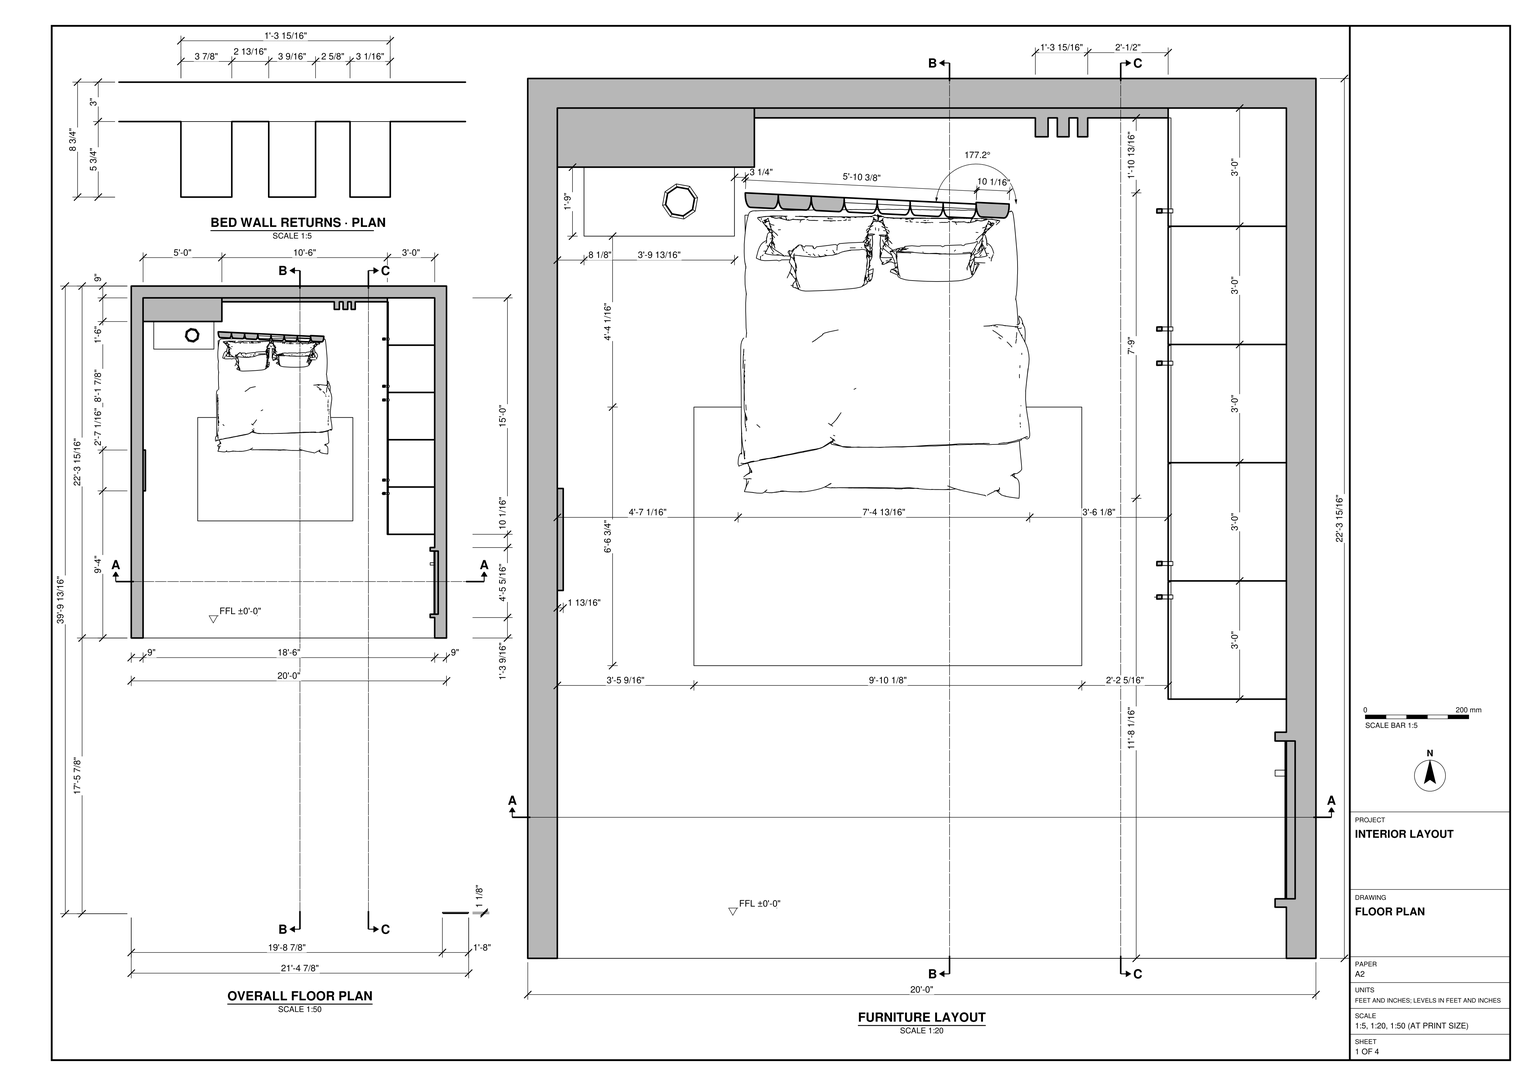
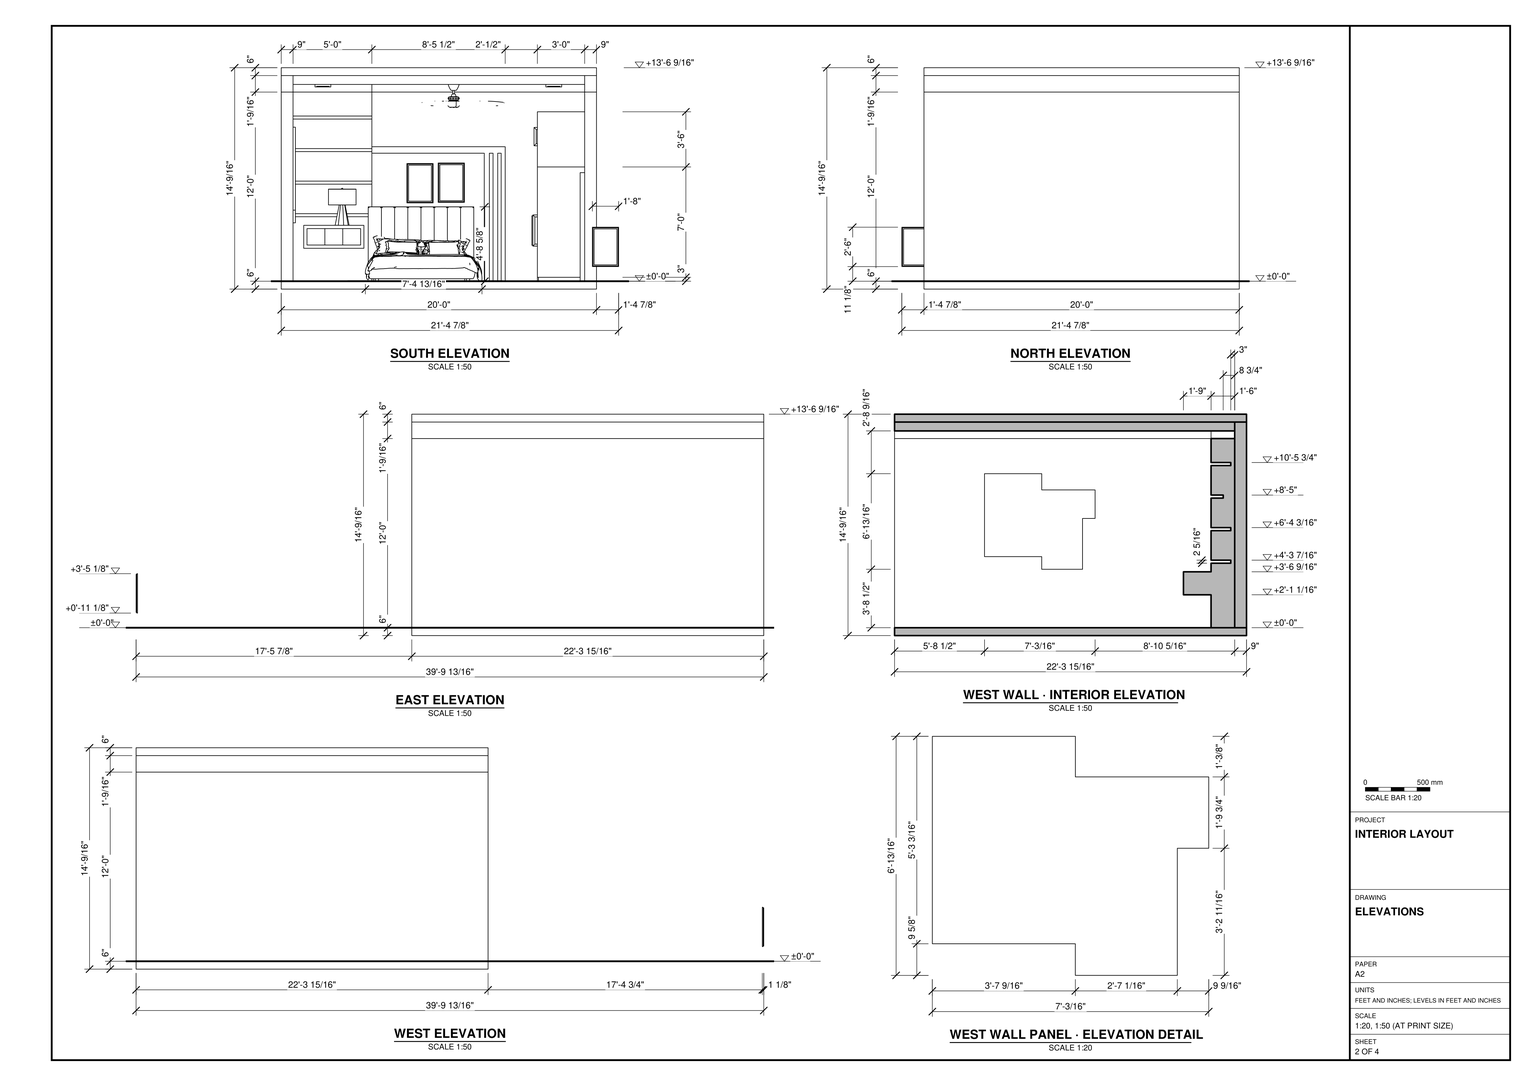
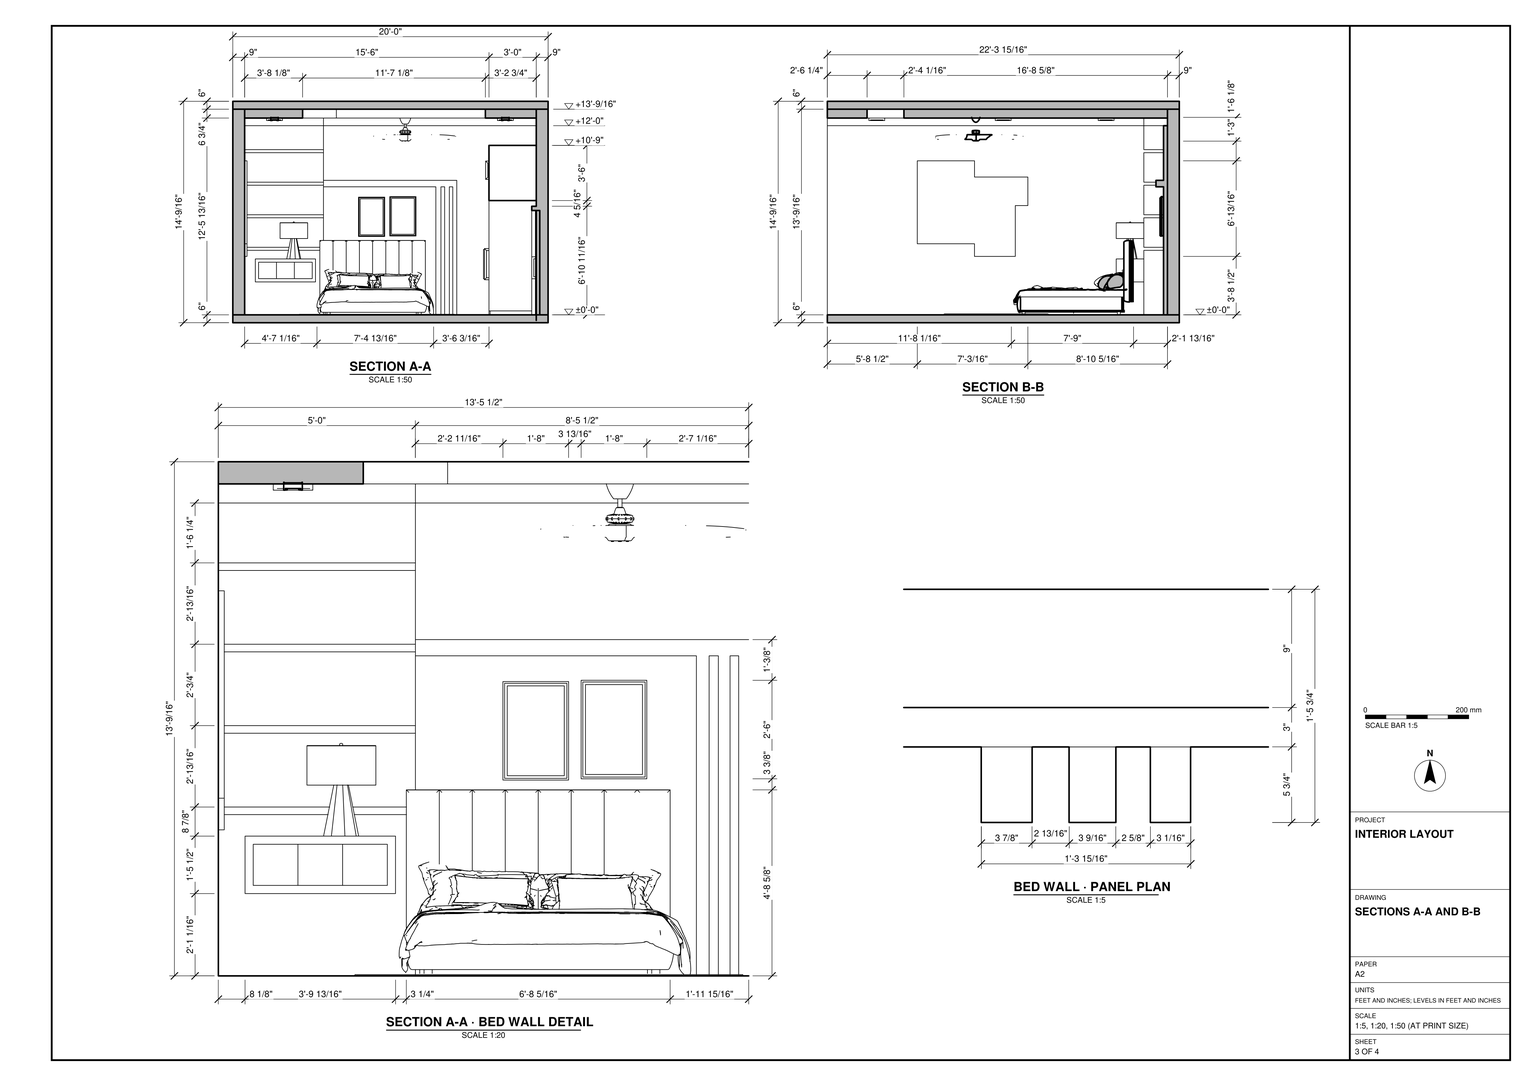
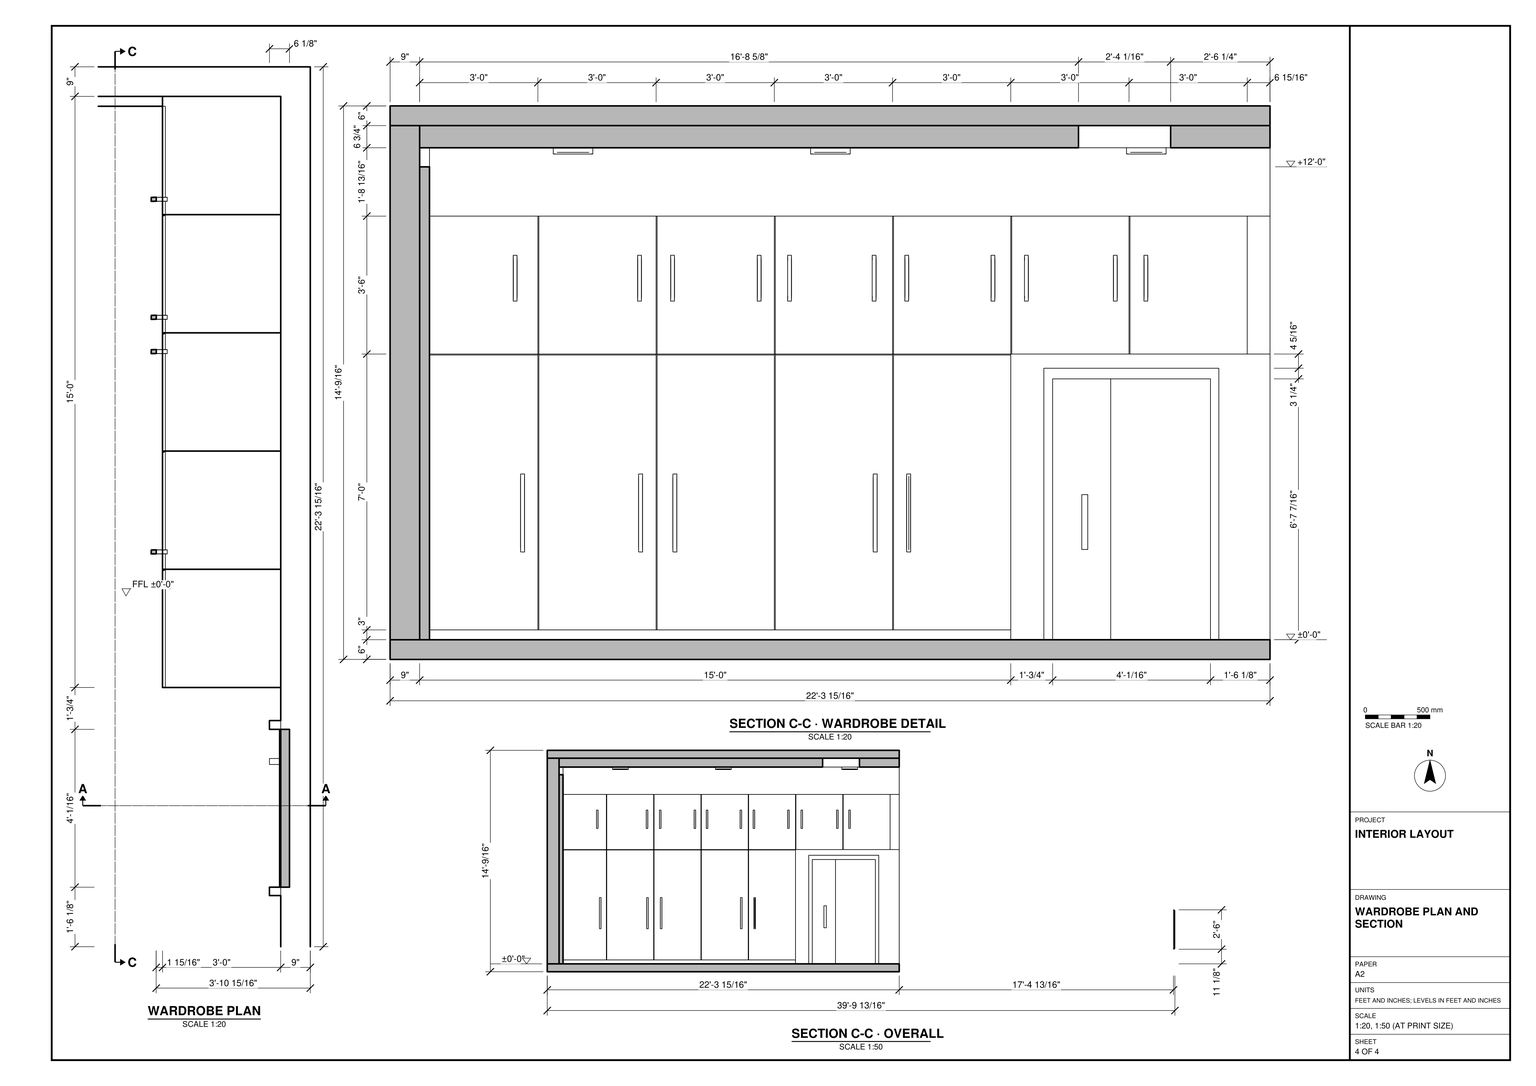
Build the bedroom interior in SketchUp using the four sheets in task_files/diagram_01.pdf. Work in feet and inches, with the finished floor at ±0'-0". The complete layout measures 21'-4 7/8" in width, 39'-9 13/16" in depth and 14'-9/16" in height. Use the overall plan to position elements outside the room; do not stretch the room shell to match those overall dimensions.

Form the three-sided shell with 9" walls and leave the south end open as drawn. Model the floor slab, overhead slab and stepped ceiling profile from the sections. Place the bed against the north wall at the slight angle shown in the furniture plan. Distinguish the divided headboard from the wall panel behind it, including the projecting vertical returns to the right. Fit the floating bedside cabinet and shelves to the left of the bed. Run the tall wardrobe along the east wall, matching its depth and bay divisions, and locate the stepped wall panel on the west wall. Place the rug beneath the foot of the bed, the lamp on the bedside cabinet, the pictures above the headboard and the fan and lights at ceiling level.

Decor and loose items may be any suitable library components. Keep shell elements and individual furniture and joinery pieces in separate groups or components, and use components for repeated parts. Save one SketchUp model as output_files/bedroom_interior_with_its_fitted_bed_wall_and_wardrobe.skp.

# SketchUp Ruby script. Lengths in inches.
U = 1.inch
M = Sketchup.active_model
def pt(a) = Geom::Point3d.new(a.map { |v| v * U })
def face(e, loops, mat)
  f = e.add_face(loops[0].map { |a| pt(a) })
  loops[1..].each { |l| e.add_face(l.map { |a| pt(a) }).erase! }
  f.material = f.back_material = mat if mat
  f
end
# faces: each face lists its corners as indices into pts; further lists are holes
def faces(e, pts, list, mat = nil) = list.each { |f| face(e, (f[0].is_a?(Array) ? f : [f]).map { |l| l.map { |i| pts[i] } }, mat) }
# xy, xz, yz: faces in a plane at the given z, y or x. An outline is a flat list of corners, or four numbers for a rectangle; further outlines are holes
def ring(l) = l.size == 4 ? [[l[0], l[1]], [l[2], l[1]], [l[2], l[3]], [l[0], l[3]]] : l.each_slice(2).to_a
def flat(e, list, mat, &to3) = list.each { |f| face(e, (f[0].is_a?(Array) ? f : [f]).map { |l| ring(l).map { |u, v| to3.(u, v) } }, mat) }
def xy(e, z, list, mat = nil) = flat(e, list, mat) { |x, y| [x, y, z] }
def xz(e, y, list, mat = nil) = flat(e, list, mat) { |x, z| [x, y, z] }
def yz(e, x, list, mat = nil) = flat(e, list, mat) { |y, z| [x, y, z] }
def lines(e, pts, list) = list.each { |a, b| e.add_line(pt(pts[a]), pt(pts[b])) }
# prism: a flat outline (further loops are holes) pulled along v
def prism(e, loops, v, mat = nil)
  f = face(e, loops, mat); d = Geom::Vector3d.new(v.map { |x| x * U })
  f.pushpull(f.normal.samedirection?(d) ? d.length : -d.length)
end
def box(e, o, s, mat = nil) = prism(e, [[o, [o[0] + s[0], o[1], o[2]], [o[0] + s[0], o[1] + s[1], o[2]], [o[0], o[1] + s[1], o[2]]]], [0, 0, s[2]], mat)
def at(x, y, z, deg = 0) = Geom::Transformation.translation(pt([x, y, z])) * Geom::Transformation.rotation(ORIGIN, Z_AXIS, deg.degrees)
def axes(o, x, y, z) = Geom::Transformation.new([*x, 0, *y, 0, *z, 0, *pt(o).to_a, 1])
def part(name) = M.definitions.add(name)
# library, detail: a bought-in or finely detailed component or shape, given as its bounding box
def library(name, o, s) = part(name).tap { |d| box(d.entities, o, s) }
def detail(e, o, s) = box(e.add_group.entities, o, s)
def put(e, d, t, mat = nil) = e.add_instance(d, t).tap { |i| i.material = mat if mat }
def group(e, t, mat = nil) = e.add_group.tap { |g| g.transformation = t; g.material = mat if mat }.entities
root = M.entities
M.materials.add("3_eeeee333110148").color = [179, 176, 174]
M.materials.add("Generic").color = [237, 208, 190]
M.materials.add("[Carrera Marble]").color = [207, 207, 207]
M.materials.add("[Color M07]").color = [58, 58, 58]
M.materials.add("[Tile Limestone Large]").color = [236, 249, 228]
M.materials.add("[Upholstery Striped Multi-Colored]").color = [119, 52, 52]
M.materials.add("[Wood Cherry Original]").color = [152, 86, 42]
c1 = part("DDR842RVS01100X")
xy(c1.entities,0,[[-70.87,0,47.24,78.74]])
xy(c1.entities,0.39,[[-70.87,0,47.24,78.74]],"[Upholstery Striped Multi-Colored]")
xz(c1.entities,0,[[-70.87,0,47.24,0.39]])
xz(c1.entities,78.74,[[-70.87,0,47.24,0.39]])
yz(c1.entities,-70.87,[[0,0,78.74,0.39]])
yz(c1.entities,47.24,[[0,0,78.74,0.39]])
c2 = library("Tlon Light 450 Ceiling 152 006",[-8.86,-8.86,-3.78],[17.72,17.72,3.56])
c3 = part("Wall frame decoration")
xy(c3.entities,-6.93,[[-0.45,31.33,0.84,53.67]],"[Wood Cherry Original]")
xy(c3.entities,0,[[-0.45,0,0.84,31.33]],"[Wood Cherry Original]")
xy(c3.entities,20.92,[[-0.45,53.67,0.84,60.55]],"[Wood Cherry Original]")
xy(c3.entities,36.56,[[-0.45,31.34,0.84,60.55]],"[Wood Cherry Original]")
xy(c3.entities,45.44,[[-0.45,0,0.84,31.34]],"[Wood Cherry Original]")
xz(c3.entities,0,[[-0.45,0,0.84,45.44]],"[Wood Cherry Original]")
xz(c3.entities,31.33,[[-0.45,-6.93,0.84,0]],"[Wood Cherry Original]")
xz(c3.entities,31.34,[[-0.45,36.56,0.84,45.44]],"3_eeeee333110148")
xz(c3.entities,53.67,[[-0.45,-6.93,0.84,20.92]],"3_eeeee333110148")
xz(c3.entities,60.55,[[-0.45,20.92,0.84,36.56]],"3_eeeee333110148")
yz(c3.entities,-0.45,[[31.33,-6.93,31.33,0,0,0,0,45.44,31.34,45.44,31.34,36.56,60.55,36.56,60.55,20.92,53.67,20.92,53.67,-6.93]],"3_eeeee333110148")
yz(c3.entities,0.84,[[31.33,-6.93,53.67,-6.93,53.67,20.92,60.55,20.92,60.55,36.56,31.34,36.56,31.34,45.44,0,45.44,0,0,31.33,0]],"3_eeeee333110148")
c4 = library("Lamp+10 (1)",[0,0,0],[16.92,16.92,22.79])
c5 = library("Avation+Styled+Ceiling+Fan_JSB",[-19.77,-29.63,-13.8125],[51.59,58.16,13.8125])
c6 = library("Group\#2",[0.46,-2.1,0],[81.3,95.2,56.66])
c7 = part("Group\#5")
xy(c7.entities,1.63,[[1.63,0,2.54,1.15]])
xy(c7.entities,12.33,[[1.63,0,2.54,1.15]])
xy(c7.entities,13.96,[[0,0.06,2.54,1.21]])
yz(c7.entities,0,[[0.06,0,1.21,13.96]])
p = [[1.63,0,12.33],[0,0.06,13.96],[0,0.06,0],[1.63,0,1.63],[2.54,0.06,0],[2.54,0,1.63],
  [0,1.21,0],[1.63,1.15,1.63],[2.54,1.15,1.63],[2.54,1.21,0],[0,1.21,13.96],[1.63,1.15,12.33],
  [2.54,0,12.33],[2.54,0.06,13.96],[2.54,1.21,13.96],[2.54,1.15,12.33]]
faces(c7.entities,p,[[0,1,2,3],[3,2,4,5],[6,7,8,9],[10,11,7,6],[12,13,1,0],[14,15,11,10]])
c8 = part("Group\#6")
p = [[1.53,0.04,1.53],[0,0,0],[4.89,0,0],[4.89,0.04,1.53],[0,0,23.78],[0.03,1.21,23.75],
  [0.03,1.21,0.03],[4.89,1.21,0.03],[1.53,0.04,22.24],[1.5625,1.25,22.21],[1.5625,1.25,1.5625],[4.89,1.25,1.5625],
  [4.89,0.04,22.24],[4.89,0,23.78],[4.89,1.25,22.21],[4.89,1.21,23.75]]
faces(c8.entities,p,[[0,1,2,3],[4,5,6,1],[1,6,7,2],[8,4,1,0],[5,9,10,6],[6,10,11,7],[9,8,0,10],[10,0,3,11],
  [12,13,4,8],[14,12,8,9],[15,14,9,5],[13,15,5,4]])
xy(root,-6,[[0,209.88,240,477.82]])
xy(root,0,[[0,209.88,9,209.88,9,468.82,231,468.82,231,209.88,240,209.88,240,477.82,0,477.82],[227.5625,225.46,231,228.01],[227.5625,276.07,231,278.75],[195.86,288.82,231,288.82,231,468.82,195,468.82,195,465.82,195.86,465.82],[9,450.82,69,468.82],
  [69,465.82,195,468.82]])
xy(root,0,[[9,209.88,231,209.88,231,225.46,227.5625,225.46,227.5625,228.01,231,228.01,231,276.07,227.5625,276.07,227.5625,278.75,231,278.75,231,288.82,195.86,288.82,195.86,465.82,170.5,465.82,170.5,460.07,167.4375,460.07,167.4375,465.82,164.8125,465.82,164.8125,460.07,161.25,460.07,161.25,465.82,158.4375,465.82,158.4375,460.07,154.5625,460.07,154.5625,465.82,69,465.82,69,450.82,9,450.82]],"[Tile Limestone Large]")
xy(root,3,[[195,288.82,195.86,324.52],[195.86,288.82,231,324.82],[195.3,324.52,195.86,324.82],[195,324.82,195.86,360.52],[195.86,324.82,231,360.82],
  [195.3,360.52,195.86,360.82],[195,360.82,195.86,396.52],[195.86,360.82,231,396.82],[195.3,396.52,195.86,396.82],[195,396.82,195.86,432.52],
  [195.86,396.82,231,432.82],[195.3,432.52,195.86,432.82],[195,432.82,195.86,465.82],[195.86,432.82,231,432.82,231,468.82,195,468.82,195,465.82,195.86,465.82]])
xy(root,25.0625,[[17.13,429.8,62.94,450.82]])
xy(root,42.5625,[[17.13,429.8,62.94,450.82]],"[Wood Cherry Original]")
xy(root,49.11,[[9,450.82,69,465.82]],"[Wood Cherry Original]")
xy(root,51.42,[[9,450.82,69,465.82]],"[Wood Cherry Original]")
xy(root,73.89,[[9,450.82,69,465.82]],"[Wood Cherry Original]")
xy(root,76.2,[[9,450.82,69,465.82]],"[Wood Cherry Original]")
xy(root,79.4375,[[227.5625,228.01,231,276.07]])
xy(root,82.67,[[227.5625,225.46,231,278.75]])
xy(root,86.7,[[195,324.82,195.3,360.52],[195,360.82,195.3,396.52],[195,396.82,195.3,432.52],[195,432.82,195.3,465.82]])
xy(root,87,[[195,288.82,231,288.82,231,324.82,195.3,324.82,195.3,324.52,195,324.52],[195,324.82,195.3,360.52],[195.3,324.82,231,360.82],[195,360.52,195.3,360.82],[195,360.82,195.3,396.52],
  [195.3,360.82,231,396.82],[195,396.82,195.3,432.52],[195.3,396.82,231,432.82],[195,432.82,195.3,465.82],[195.3,432.82,231,432.82,231,468.82,195,468.82,195,465.82,195.3,465.82]])
xy(root,87,[[195,216.82,195,252.52,195.3,252.52,195.3,252.82,231,252.82,231,216.82],[195,252.82,195,288.52,195.3,288.52,195.3,288.82,231,288.82,231,252.82]],"[Wood Cherry Original]")
xy(root,97.46,[[69,460.07,154.5625,465.82],[158.4375,460.07,161.25,465.82],[164.8125,460.07,167.4375,465.82]],"[Wood Cherry Original]")
xy(root,98.67,[[9,450.82,69,460.07]],"[Wood Cherry Original]")
xy(root,100.99,[[9,450.82,69,460.07]],"[Wood Cherry Original]")
xy(root,102.4,[[69,460.07,170.5,465.82]],"[Wood Cherry Original]")
xy(root,103.12,[[192.46,439.18,195,440.33]])
xy(root,123.46,[[9,450.82,69,465.82]],"[Wood Cherry Original]")
xy(root,125.77,[[9,450.82,69,465.82]],"[Wood Cherry Original]")
xy(root,129,[[195,465.82,231,468.82]])
xy(root,129,[[195,216.82,231,216.82,231,252.82,195.3,252.82,195.3,252.52,195,252.52],[195,252.82,231,252.82,231,288.82,195.3,288.82,195.3,288.52,195,288.52],[195,288.82,231,288.82,231,324.82,195.3,324.82,195.3,324.52,195,324.52],[195,324.82,231,360.82],[195,360.82,231,360.82,231,396.82,195.3,396.82,195.3,396.52,195,396.52],
  [195,396.82,231,396.82,231,432.82,195.3,432.82,195.3,432.52,195,432.52],[195,432.82,231,465.82]],"[Wood Cherry Original]")
xy(root,144,[[69,465.82,231,468.82]])
xy(root,144,[[9,450.82,69,468.82]],"[Wood Cherry Original]")
xy(root,149.8125,[[[9,209.88,231,468.82],[53.125,240.14,192.26,240.14,192.26,268.2,78.8125,268.2,78.8125,438.76,53.125,438.76]]],"Generic")
xy(root,156.5625,[[0,209.88,0,477.82,240,477.82,240,209.88,231,209.88,231,468.82,9,468.82,9,209.88],[[9,209.88,231,468.82],[53.125,240.14,53.125,438.76,78.8125,438.76,78.8125,268.2,192.26,268.2,192.26,240.14]]])
xy(root,156.5625,[[53.125,240.14,53.125,438.76,78.8125,438.76,78.8125,268.2,192.26,268.2,192.26,240.14]],"[Wood Cherry Original]")
xy(root,162.5625,[[0,209.88,240,477.82]])
xz(root,209.88,[[0,-6,240,0],[0,0,9,144],[231,0,240,144],[0,144,9,156.5625],[231,144,240,156.5625],
  [9,149.8125,231,156.5625],[0,156.5625,240,162.5625]])
xz(root,216.82,[[195,87,231,129]],"[Wood Cherry Original]")
xz(root,225.46,[[227.5625,0,231,82.67]],"Generic")
xz(root,228.01,[[227.5625,0,231,79.4375]])
xz(root,240.14,[[53.125,149.8125,192.26,156.5625]])
xz(root,252.52,[[195,87,195.3,129]])
xz(root,252.82,[[195,87,195.3,129],[195.3,87,231,129]])
xz(root,268.2,[[78.8125,149.8125,192.26,156.5625]],"Generic")
xz(root,276.07,[[227.5625,0,231,79.4375]],"Generic")
xz(root,278.75,[[227.5625,0,231,82.67]],"Generic")
xz(root,288.52,[[195,87,195.3,129]])
xz(root,288.82,[[195,87,195.3,129],[195.3,87,231,129]])
xz(root,288.82,[[195.86,0,231,3],[195,3,231,87]],"[Wood Cherry Original]")
xz(root,324.52,[[195,3,195.3,86.7],[195,86.7,195.3,87],[195,87,195.3,129]])
xz(root,324.82,[[195,3,195.3,86.7],[195.3,3,231,87],[195,87,195.3,129],[195.3,87,231,129]])
xz(root,360.52,[[195,3,195.3,86.7]])
xz(root,360.82,[[195,3,195.3,86.7],[195.3,3,231,87],[195,87,231,129]])
xz(root,396.52,[[195,3,195.3,86.7],[195,87,195.3,129]])
xz(root,396.82,[[195,3,195.3,86.7],[195.3,3,231,87],[195,87,195.3,129],[195.3,87,231,129]])
xz(root,429.8,[[19.62,27.55,33.23,40.07],[33.23,27.55,46.84,40.07],[46.84,27.55,60.45,40.07]])
xz(root,429.8,[[[17.13,25.0625,62.94,42.5625],[19.62,27.55,60.45,40.07]]],"[Wood Cherry Original]")
xz(root,432.52,[[195,3,195.3,86.7],[195,87,195.3,129]])
xz(root,432.82,[[195,3,195.3,86.7],[195.3,3,231,87],[195,87,195.3,129],[195.3,87,231,129]])
xz(root,438.76,[[53.125,149.8125,78.8125,156.5625]],"Generic")
xz(root,450.82,[[[9,0,69,49.11],[17.13,25.0625,62.94,42.5625]],[9,51.42,69,73.89],[9,76.2,69,98.67],[9,100.99,69,123.46],[9,125.77,69,144]],"[Wood Cherry Original]")
xz(root,460.07,[[9,98.67,69,100.99]])
xz(root,460.07,[[154.5625,0,158.4375,0,158.4375,97.46,161.25,97.46,161.25,0,164.8125,0,164.8125,97.46,167.4375,97.46,167.4375,0,170.5,0,170.5,102.4,69,102.4,69,97.46,154.5625,97.46]],"[Wood Cherry Original]")
xz(root,465.82,[[158.4375,0,161.25,97.46],[164.8125,0,167.4375,97.46],[195,0,195.86,3],[9,49.11,69,51.42],[9,73.89,69,76.2],
  [195,86.7,195.3,87],[9,123.46,69,125.77]])
xz(root,465.82,[[170.5,0,195,0,195,129,231,129,231,144,69,144,69,102.4,170.5,102.4],[69,0,154.5625,97.46]],"Generic")
xz(root,468.82,[[9,0,69,144],[69,0,69,144,231,144,231,129,195,129,195,0],[195,0,231,3],[195,3,231,87],[195,87,231,129],
  [9,144,69,149.8125],[69,144,231,149.8125],[9,149.8125,69,156.5625],[69,149.8125,231,156.5625]])
xz(root,477.82,[[0,-6,240,0],[0,0,240,144],[0,144,240,156.5625],[0,156.5625,240,162.5625]])
yz(root,0,[[209.88,-6,477.82,0],[209.88,0,477.82,144],[209.88,144,477.82,156.5625],[209.88,156.5625,477.82,162.5625]])
yz(root,9,[[450.82,0,468.82,0,468.82,144,450.82,144,450.82,125.77,465.82,125.77,465.82,123.46,450.82,123.46,450.82,100.99,460.07,100.99,460.07,98.67,450.82,98.67,450.82,76.2,465.82,76.2,465.82,73.89,450.82,73.89,450.82,51.42,465.82,51.42,465.82,49.11,450.82,49.11],[450.82,144,468.82,149.8125],[209.88,149.8125,450.82,156.5625],[450.82,149.8125,468.82,156.5625]])
yz(root,9,[[209.88,0,450.82,0,450.82,49.11,465.82,49.11,465.82,51.42,450.82,51.42,450.82,73.89,465.82,73.89,465.82,76.2,450.82,76.2,450.82,98.67,460.07,98.67,460.07,100.99,450.82,100.99,450.82,123.46,465.82,123.46,465.82,125.77,450.82,125.77,450.82,144,209.88,144],[209.88,144,450.82,149.8125]],"Generic")
yz(root,17.13,[[429.8,25.0625,450.82,42.5625]],"[Wood Cherry Original]")
yz(root,53.125,[[240.14,149.8125,438.76,156.5625]],"Generic")
yz(root,62.94,[[429.8,25.0625,450.82,42.5625]],"[Wood Cherry Original]")
yz(root,69,[[465.82,0,468.82,0,468.82,144,465.82,144,465.82,102.4,460.07,102.4,460.07,97.46,465.82,97.46]])
yz(root,69,[[450.82,0,465.82,49.11],[450.82,51.42,465.82,73.89],[450.82,76.2,465.82,76.2,465.82,97.46,460.07,97.46,460.07,98.67,450.82,98.67],[450.82,100.99,460.07,100.99,460.07,102.4,465.82,102.4,465.82,123.46,450.82,123.46],[450.82,125.77,465.82,144]],"[Wood Cherry Original]")
yz(root,78.8125,[[268.2,149.8125,438.76,156.5625]])
yz(root,154.5625,[[460.07,0,465.82,97.46]],"[Wood Cherry Original]")
yz(root,158.4375,[[460.07,0,465.82,97.46]],"[Wood Cherry Original]")
yz(root,161.25,[[460.07,0,465.82,97.46]],"[Wood Cherry Original]")
yz(root,164.8125,[[460.07,0,465.82,97.46]],"[Wood Cherry Original]")
yz(root,167.4375,[[460.07,0,465.82,97.46]],"[Wood Cherry Original]")
yz(root,170.5,[[460.07,0,465.82,102.4]],"[Wood Cherry Original]")
yz(root,192.26,[[240.14,149.8125,268.2,156.5625]])
yz(root,194.09,[[439.125,104.75,440.28,115.45]])
yz(root,195,[[465.82,0,468.82,3],[465.82,3,468.82,87],[320.56,48.93,320.52,50.46,319.31,50.49,319.34,48.96],[288.82,86.7,324.52,87],[360.52,87,360.82,129],
  [465.82,87,468.82,129],[439.125,115.45,440.28,115.45,440.33,117.08,439.18,117.08]])
yz(root,195,[[[288.82,3,324.52,86.7],[320.56,48.93,320.52,50.46,319.31,50.49,319.34,48.96],[319.31,26.71,320.52,26.74,320.56,28.27,319.34,28.25]],[324.82,3,360.52,86.7],[360.82,3,396.52,86.7],[396.82,3,432.52,86.7],[432.82,3,465.82,86.7]],"[Carrera Marble]")
yz(root,195,[[216.82,87,252.52,129],[252.82,87,288.52,129],[288.82,87,324.52,129],[324.82,87,360.52,129],[360.82,87,396.52,129],
  [396.82,87,432.52,129],[[432.82,87,465.82,129],[439.18,103.12,440.33,103.12,440.28,104.75,439.125,104.75],[439.125,115.45,440.28,115.45,440.33,117.08,439.18,117.08]]],"[Wood Cherry Original]")
yz(root,195.3,[[324.52,3,324.82,87],[360.52,3,360.82,87],[396.52,3,396.82,87],[432.52,3,432.82,87],[324.82,86.7,360.52,87],
  [360.82,86.7,396.52,87],[396.82,86.7,432.52,87],[432.82,86.7,465.82,87],[252.52,87,252.82,129],[288.52,87,288.82,129],
  [324.52,87,324.82,129],[396.52,87,396.82,129],[432.52,87,432.82,129]])
yz(root,195.86,[[288.82,0,465.82,3]],"[Wood Cherry Original]")
yz(root,227.5625,[[225.46,0,225.46,82.67,278.75,82.67,278.75,0,276.07,0,276.07,79.4375,228.01,79.4375,228.01,0]],"Generic")
yz(root,231,[[223.78,-4.24,280.31,0],[228.01,0,276.07,79.4375],[288.82,0,468.82,3],[288.82,3,324.82,87],[324.82,3,360.82,87],
  [360.82,3,396.82,87],[396.82,3,432.82,87],[432.82,3,468.82,87],[216.82,87,252.82,129],[252.82,87,288.82,129],
  [288.82,87,324.82,129],[324.82,87,360.82,129],[360.82,87,396.82,129],[396.82,87,432.82,129],[432.82,87,468.82,129],
  [465.82,129,468.82,144],[465.82,144,468.82,149.8125],[209.88,149.8125,465.82,156.5625],[465.82,149.8125,468.82,156.5625]])
yz(root,231,[[209.88,0,209.88,87,288.82,87,288.82,0,278.75,0,278.75,82.67,225.46,82.67,225.46,0],[209.88,87,216.82,129],[209.88,129,465.82,149.8125]],"Generic")
yz(root,240,[[209.88,-6,477.82,0],[209.88,0,477.82,144],[209.88,144,477.82,156.5625],[209.88,156.5625,477.82,162.5625]])
p = [[195,439.49,116.47],[193.0625,439.49,116.47],[193.0625,439.49,103.72],[195,439.49,103.72],[195,319.88,49.79],[190.8125,319.88,49.79],
  [190.8125,319.88,27.41],[195,319.88,27.41]]
lines(root,p,[[0,1],[1,2],[2,3],[4,5],[5,6],[6,7]])
put(root,c1,at(121.46,299.02,0))
put(root,c2,axes([207.48,247.55,150.48],[0.68,0,0],[0,0.68,0],[0,0,0.68]))
put(root,c2,axes([207.48,343.74,150.48],[0.68,0,0],[0,0.68,0],[0,0,0.68]))
put(root,c2,axes([207.48,422.12,150.48],[0.68,0,0],[0,0.68,0],[0,0,0.68]))
put(root,c2,axes([31.73,343.74,150.48],[0.68,0,0],[0,0.68,0],[0,0,0.68]))
put(root,c2,axes([31.73,422.12,150.48],[0.68,0,0],[0,0.68,0],[0,0,0.68]))
put(root,c2,axes([31.73,247.55,150.48],[0.68,0,0],[0,0.68,0],[0,0,0.68]))
put(root,c3,axes([9.63,278.37,54.1],[1.39,0,0],[0,1.39,0],[0,0,1.39]))
put(root,c4,axes([35.97,429.8,42.5625],[1.24,0,0],[0,1.24,0],[0,0,1.24]))
put(root,c5,axes([131.27,322.93,150.34],[1.31,0,0],[0,1.31,0],[0,0,1.31]))
g1 = group(root,at(227.5625,228.01,0))
xy(g1,0,[[3.11,0,6.11,48.0625]],"[Wood Cherry Original]")
xy(g1,27.48,[[0,37.36,3.11,39.1875]],"[Wood Cherry Original]")
xy(g1,29.01,[[1.52,37.36,3.11,39.1875]],"[Color M07]")
xy(g1,42.67,[[1.52,37.36,3.11,39.1875]],"[Color M07]")
xy(g1,44.19,[[0,37.36,3.11,39.1875]],"[Color M07]")
xy(g1,79.4375,[[3.11,0,6.11,48.0625]],"[Wood Cherry Original]")
xz(g1,0,[[3.11,0,6.11,79.4375]],"[Wood Cherry Original]")
xz(g1,37.36,[[0,27.48,3.11,27.48,3.11,29.01,1.52,29.01,1.52,42.67,3.11,42.67,3.11,44.19,0,44.19]],"[Color M07]")
xz(g1,39.1875,[[0,27.48,0,44.19,3.11,44.19,3.11,42.67,1.52,42.67,1.52,29.01,3.11,29.01,3.11,27.48]],"[Color M07]")
xz(g1,48.0625,[[3.11,0,6.11,79.4375]],"[Wood Cherry Original]")
yz(g1,0,[[37.36,27.48,39.1875,44.19]],"[Color M07]")
yz(g1,1.52,[[37.36,29.01,39.1875,42.67]],"[Wood Cherry Original]")
yz(g1,3.11,[[0,0,30.375,79.4375]],"[Carrera Marble]")
yz(g1,3.11,[[[30.375,0,48.0625,79.4375],[37.36,42.67,39.1875,44.19],[37.36,27.48,39.1875,29.01]],[37.36,42.67,39.1875,44.19]],"[Wood Cherry Original]")
yz(g1,6.11,[[0,0,48.0625,79.4375]],"[Wood Cherry Original]")
p = [[3.11,38.02,43.53],[0.67,38.02,43.53],[0.67,38.02,28.15],[3.11,38.02,28.15]]
lines(g1,p,[[0,1],[1,2],[2,3]])
put(root,c6,axes([60.66,349.97,0],[1.16,0,0],[0,1,0],[0,0,1]))
g2 = group(root,at(119.46,464.73,60.02))
xy(g2,0,[[0,-0.6,20,0]])
xy(g2,0.52,[[0.52,-1.1,19.48,-0.6],[0.52,-0.6,19.48,0]])
xy(g2,1.32,[[1.32,-1.1,18.68,-0.3]])
xy(g2,28.68,[[1.32,-1.1,18.68,-0.3]])
xy(g2,29.48,[[0.52,-1.1,19.48,-0.6],[0.52,-0.6,19.48,0]])
xy(g2,30,[[0,-0.6,20,0]])
xz(g2,-1.1,[[[0.52,0.52,19.48,29.48],[1.32,1.32,18.68,28.68]]])
xz(g2,-0.6,[[[0,0,20,30],[0.52,0.52,19.48,29.48]]])
xz(g2,-0.3,[[1.32,1.32,18.68,28.68]])
xz(g2,0,[[[0,0,20,30],[0.52,0.52,19.48,29.48]]])
yz(g2,0,[[-0.6,0,0,30]])
yz(g2,0.52,[[-1.1,0.52,-0.6,29.48],[-0.6,0.52,0,29.48]])
yz(g2,1.32,[[-1.1,1.32,-0.3,28.68]])
yz(g2,18.68,[[-1.1,1.32,-0.3,28.68]])
yz(g2,19.48,[[-1.1,0.52,-0.6,29.48],[-0.6,0.52,0,29.48]])
yz(g2,20,[[-0.6,0,0,30]])
g3 = group(root,at(236.86,1.1,11.14))
xy(g3,0,[[0,-0.6,20,0]])
xy(g3,0.52,[[0.52,-1.1,19.48,-0.6],[0.52,-0.6,19.48,0]])
xy(g3,1.32,[[1.32,-1.1,18.68,-0.3]])
xy(g3,28.68,[[1.32,-1.1,18.68,-0.3]])
xy(g3,29.48,[[0.52,-1.1,19.48,-0.6],[0.52,-0.6,19.48,0]])
xy(g3,30,[[0,-0.6,20,0]])
xz(g3,-1.1,[[[0.52,0.52,19.48,29.48],[1.32,1.32,18.68,28.68]]])
xz(g3,-0.6,[[[0,0,20,30],[0.52,0.52,19.48,29.48]]])
xz(g3,-0.3,[[1.32,1.32,18.68,28.68]])
xz(g3,0,[[[0,0,20,30],[0.52,0.52,19.48,29.48]]])
yz(g3,0,[[-0.6,0,0,30]])
yz(g3,0.52,[[-1.1,0.52,-0.6,29.48],[-0.6,0.52,0,29.48]])
yz(g3,1.32,[[-1.1,1.32,-0.3,28.68]])
yz(g3,18.68,[[-1.1,1.32,-0.3,28.68]])
yz(g3,19.48,[[-1.1,0.52,-0.6,29.48],[-0.6,0.52,0,29.48]])
yz(g3,20,[[-0.6,0,0,30]])
g4 = group(root,at(115.65,463.92,59.63))
xy(g4,0,[[-20,-0.6,0,0]])
xy(g4,0.52,[[-19.48,-1.1,-0.52,-0.6],[-19.48,-0.6,-0.52,0]])
xy(g4,1.32,[[-18.68,-1.1,-1.32,-0.3]])
xy(g4,28.68,[[-18.68,-1.1,-1.32,-0.3]])
xy(g4,29.48,[[-19.48,-1.1,-0.52,-0.6],[-19.48,-0.6,-0.52,0]])
xy(g4,30,[[-20,-0.6,0,0]])
xz(g4,-1.1,[[[-19.48,0.52,-0.52,29.48],[-18.68,1.32,-1.32,28.68]]])
xz(g4,-0.6,[[[-20,0,0,30],[-19.48,0.52,-0.52,29.48]]])
xz(g4,-0.3,[[-18.68,1.32,-1.32,28.68]])
xz(g4,0,[[[-20,0,0,30],[-19.48,0.52,-0.52,29.48]]])
yz(g4,-20,[[-0.6,0,0,30]])
yz(g4,-19.48,[[-1.1,0.52,-0.6,29.48],[-0.6,0.52,0,29.48]])
yz(g4,-18.68,[[-1.1,1.32,-0.3,28.68]])
yz(g4,-1.32,[[-1.1,1.32,-0.3,28.68]])
yz(g4,-0.52,[[-1.1,0.52,-0.6,29.48],[-0.6,0.52,0,29.48]])
yz(g4,0,[[-0.6,0,0,30]])
g5 = group(root,at(192.46,439.18,103.12))
p = [[0,0,13.96],[0,0,0]]
lines(g5,p,[[0,1]])
put(root,c7,at(192.46,439.125,103.12),"[Color M07]")
put(root,c7,at(192.46,401.25,103.12),"[Color M07]")
put(root,c7,at(192.46,391.1875,103.12),"[Color M07]")
put(root,c7,at(192.46,364.8125,103.12),"[Color M07]")
put(root,c7,at(192.46,355.5625,103.12),"[Color M07]")
put(root,c7,at(192.46,329.8125,103.12),"[Color M07]")
put(root,c7,at(192.46,319.875,103.12),"[Color M07]")
put(root,c7,at(192.46,293.625,103.12),"[Color M07]")
put(root,c7,at(192.46,283.4375,103.12),"[Color M07]")
put(root,c7,at(192.46,256.375,103.12),"[Color M07]")
put(root,c7,at(192.46,247.0625,103.12),"[Color M07]")
put(root,c8,at(191.55,319.31,26.71),"[Color M07]")
put(root,c8,at(191.55,329.49,26.71),"[Color M07]")
put(root,c8,at(191.55,390.49,26.71),"[Color M07]")
put(root,c8,at(191.55,400.93,26.71),"[Color M07]")
put(root,c8,at(191.55,436.87,26.71),"[Color M07]")
